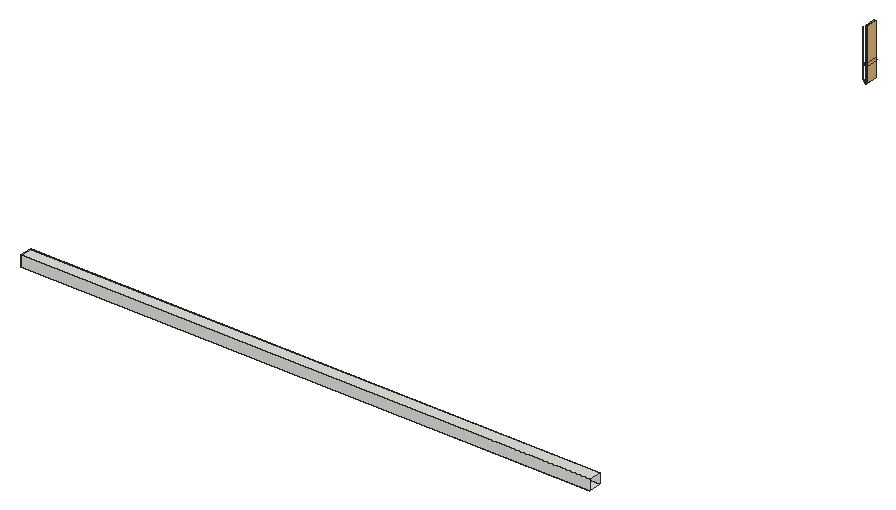
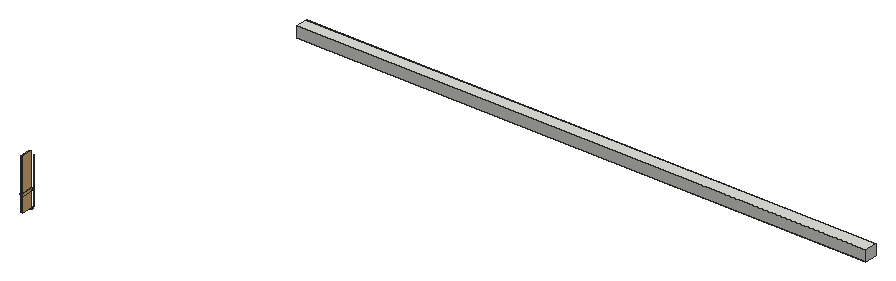
# SketchUp Ruby script. Lengths in inches.
U = 1.inch
M = Sketchup.active_model
def pt(a) = Geom::Point3d.new(a.map { |v| v * U })
def face(e, loops, mat)
  f = e.add_face(loops[0].map { |a| pt(a) })
  loops[1..].each { |l| e.add_face(l.map { |a| pt(a) }).erase! }
  f.material = f.back_material = mat if mat
  f
end
# faces: each face lists its corners as indices into pts; further lists are holes
def faces(e, pts, list, mat = nil) = list.each { |f| face(e, (f[0].is_a?(Array) ? f : [f]).map { |l| l.map { |i| pts[i] } }, mat) }
# xy, xz, yz: faces in a plane at the given z, y or x. An outline is a flat list of corners, or four numbers for a rectangle; further outlines are holes
def ring(l) = l.size == 4 ? [[l[0], l[1]], [l[2], l[1]], [l[2], l[3]], [l[0], l[3]]] : l.each_slice(2).to_a
def flat(e, list, mat, &to3) = list.each { |f| face(e, (f[0].is_a?(Array) ? f : [f]).map { |l| ring(l).map { |u, v| to3.(u, v) } }, mat) }
def xy(e, z, list, mat = nil) = flat(e, list, mat) { |x, y| [x, y, z] }
def xz(e, y, list, mat = nil) = flat(e, list, mat) { |x, z| [x, y, z] }
def yz(e, x, list, mat = nil) = flat(e, list, mat) { |y, z| [x, y, z] }
def lines(e, pts, list) = list.each { |a, b| e.add_line(pt(pts[a]), pt(pts[b])) }
# prism: a flat outline (further loops are holes) pulled along v
def prism(e, loops, v, mat = nil)
  f = face(e, loops, mat); d = Geom::Vector3d.new(v.map { |x| x * U })
  f.pushpull(f.normal.samedirection?(d) ? d.length : -d.length)
end
def box(e, o, s, mat = nil) = prism(e, [[o, [o[0] + s[0], o[1], o[2]], [o[0] + s[0], o[1] + s[1], o[2]], [o[0], o[1] + s[1], o[2]]]], [0, 0, s[2]], mat)
def at(x, y, z, deg = 0) = Geom::Transformation.translation(pt([x, y, z])) * Geom::Transformation.rotation(ORIGIN, Z_AXIS, deg.degrees)
def axes(o, x, y, z) = Geom::Transformation.new([*x, 0, *y, 0, *z, 0, *pt(o).to_a, 1])
def part(name) = M.definitions.add(name)
# library, detail: a bought-in or finely detailed component or shape, given as its bounding box
def library(name, o, s) = part(name).tap { |d| box(d.entities, o, s) }
def detail(e, o, s) = box(e.add_group.entities, o, s)
def put(e, d, t, mat = nil) = e.add_instance(d, t).tap { |i| i.material = mat if mat }
def group(e, t, mat = nil) = e.add_group.tap { |g| g.transformation = t; g.material = mat if mat }.entities
root = M.entities
M.materials.add("Material \#1").color = [140, 140, 140]
c1 = library("3DGeom~4_Defintion",[-18.02,-499.97,-221.16],[36.04,1000,262.12])
c2 = part("3DGeom~5_Defintion")
xy(c2.entities,-225.24,[[-0.79,-499.98,-2.33,-499.64,7.45,-496.14],[-0.79,-499.98,7.45,-496.14,1.58,-499.88],[1.58,-499.88,7.45,-496.14,3.84,-499.16],[-2.33,-499.64,7.4,-485.75,7.45,-496.14],[3.84,-499.16,7.45,-496.14,5.85,-497.89],
  [7.45,-496.14,7.4,-485.75,8.24,-487.08],[7.45,-496.14,8.24,-487.08,8.96,-489.34],[7.45,-496.14,8.96,-489.34,9.0625,-491.71],[7.45,-496.14,9.0625,-491.71,8.55,-494.03],[-7.4,-496.08,-8.24,-494.76,2.32,-482.2],
  [-8.24,-494.76,-8.96,-492.5,2.32,-482.2],[-8.96,-492.5,-9.0625,-490.125,2.32,-482.2],[-9.0625,-490.125,-8.55,-487.81,2.32,-482.2],[-8.55,-487.81,-7.45,-485.7,2.32,-482.2],[-7.45,-485.7,-5.85,-483.95,2.32,-482.2],
  [-5.85,-483.95,-3.84,-482.68,2.32,-482.2],[-3.84,-482.68,-1.58,-481.96,2.32,-482.2],[2.32,-482.2,-1.58,-481.96,0.79,-481.86],[0,481.82,-2.35,482.13,-6.92,496.71],[0,481.82,-6.92,496.71,1.55,482.04],
  [-2.35,482.13,-4.55,483.04,-6.92,496.71],[-4.55,483.04,-6.43,484.49,-6.92,496.71],[-6.43,484.49,-7.88,486.37,-6.92,496.71],[6.92,485.12,-1.55,499.8125,7.88,495.47],[6.92,485.12,7.88,495.47,7.88,486.37],
  [-7.88,486.37,-8.79,488.57,-6.92,496.71],[7.88,486.37,7.88,495.47,8.79,488.57],[-8.79,488.57,-9.1,490.92,-6.92,496.71],[8.79,488.57,7.88,495.47,9.1,490.92],[-9.1,490.92,-8.79,493.28,-6.92,496.71],
  [9.1,490.92,7.88,495.47,8.79,493.28],[-8.79,493.28,-7.88,495.47,-6.92,496.71],[7.88,495.47,-1.55,499.8125,0,500.02],[7.88,495.47,0,500.02,2.35,499.71],[7.88,495.47,2.35,499.71,4.55,498.8],
  [7.88,495.47,4.55,498.8,6.43,497.35]],"Material \#1")
xy(c2.entities,-221.57,[[-2.33,-499.64,-5.22,-498.37,7.4,-485.75],[-5.22,-498.37,-7.4,-496.08,5.22,-483.47],[-5.22,-498.37,5.22,-483.47,7.4,-485.75],[-7.4,-496.08,2.32,-482.2,5.22,-483.47],[1.55,482.04,-6.92,496.71,-4.55,498.8],
  [1.55,482.04,-4.55,498.8,4.55,483.04],[4.55,483.04,-4.55,498.8,-1.55,499.8125],[4.55,483.04,-1.55,499.8125,6.92,485.12]],"Material \#1")
xy(c2.entities,38.05,[[-2.33,-499.64,7.4,-485.75,-5.22,-498.37],[-5.22,-498.37,5.22,-483.47,-7.4,-496.08],[-5.22,-498.37,7.4,-485.75,5.22,-483.47],[-7.4,-496.08,5.22,-483.47,2.32,-482.2],[1.55,482.04,-4.55,498.8,-6.92,496.71],
  [1.55,482.04,4.55,483.04,-4.55,498.8],[4.55,483.04,-1.55,499.8125,-4.55,498.8],[4.55,483.04,6.92,485.12,-1.55,499.8125]],"Material \#1")
xy(c2.entities,41.72,[[-0.79,-499.98,7.45,-496.14,-2.33,-499.64],[-0.79,-499.98,1.58,-499.88,7.45,-496.14],[1.58,-499.88,3.84,-499.16,7.45,-496.14],[-2.33,-499.64,7.45,-496.14,7.4,-485.75],[3.84,-499.16,5.85,-497.89,7.45,-496.14],
  [7.45,-496.14,8.24,-487.08,7.4,-485.75],[7.45,-496.14,8.55,-494.03,9.0625,-491.71],[7.45,-496.14,8.96,-489.34,8.24,-487.08],[7.45,-496.14,9.0625,-491.71,8.96,-489.34],[-7.4,-496.08,2.32,-482.2,-8.24,-494.76],
  [-8.24,-494.76,2.32,-482.2,-8.96,-492.5],[-8.96,-492.5,2.32,-482.2,-9.0625,-490.125],[-9.0625,-490.125,2.32,-482.2,-8.55,-487.81],[-8.55,-487.81,2.32,-482.2,-7.45,-485.7],[-7.45,-485.7,2.32,-482.2,-5.85,-483.95],
  [-5.85,-483.95,2.32,-482.2,-3.84,-482.68],[-3.84,-482.68,2.32,-482.2,-1.58,-481.96],[2.32,-482.2,0.79,-481.86,-1.58,-481.96],[0,481.82,-6.92,496.71,-2.35,482.13],[0,481.82,1.55,482.04,-6.92,496.71],
  [-2.35,482.13,-6.92,496.71,-4.55,483.04],[-4.55,483.04,-6.92,496.71,-6.43,484.49],[-6.43,484.49,-6.92,496.71,-7.88,486.37],[6.92,485.12,7.88,495.47,-1.55,499.8125],[6.92,485.12,7.88,486.37,7.88,495.47],
  [-7.88,486.37,-6.92,496.71,-8.79,488.57],[7.88,486.37,8.79,488.57,7.88,495.47],[-8.79,488.57,-6.92,496.71,-9.1,490.92],[8.79,488.57,9.1,490.92,7.88,495.47],[-9.1,490.92,-6.92,496.71,-8.79,493.28],
  [9.1,490.92,8.79,493.28,7.88,495.47],[-8.79,493.28,-6.92,496.71,-7.88,495.47],[7.88,495.47,0,500.02,-1.55,499.8125],[7.88,495.47,2.35,499.71,0,500.02],[7.88,495.47,4.55,498.8,2.35,499.71],
  [7.88,495.47,6.43,497.35,4.55,498.8]],"Material \#1")
c3 = part("3DGeom~10_Defintion")
yz(c3.entities,-68.96,[[-797.08,-844.83,-797.08,-827.59,-922.41,-827.59],[-922.41,-844.83,-797.08,-844.83,-922.41,-827.59]],"Material \#1")
yz(c3.entities,68.97,[[-922.41,-844.83,-797.08,-827.59,-797.08,-844.83],[-922.41,-844.83,-922.41,-827.59,-797.08,-827.59],[-797.08,137.93,-922.41,155.17,-797.08,155.17],[-922.41,137.93,-922.41,155.17,-797.08,137.93]],"Material \#1")
p = [[-15.8,-989.55,-844.83],[-15.8,-989.55,-827.59],[0,-991.38,-827.59],[0,-991.38,-844.83],[15.8,-989.55,-827.59],[15.8,-989.55,-844.83],
  [-30.32,-984.36,-844.83],[-30.32,-984.36,-827.59],[30.31,-984.36,-827.59],[30.31,-984.36,-844.83],[-43.12,-976.21,-844.83],[-43.12,-976.21,-827.59],
  [43.12,-976.21,-827.59],[43.12,-976.21,-844.83],[-53.81,-965.53,-844.83],[-53.81,-965.53,-827.59],[53.8,-965.53,-827.59],[53.8,-965.53,-844.83],
  [-61.95,-952.73,-844.83],[-61.95,-952.73,-827.59],[53.8,-965.53,-827.59],[61.95,-952.73,-827.59],[61.95,-952.73,-844.83],[-67.15,-938.21,-844.83],
  [-67.15,-938.21,-827.59],[67.14,-938.21,-827.59],[67.14,-938.21,-844.83],[-68.96,-922.41,-844.83],[-68.96,-922.41,-827.59],[67.14,-938.21,-827.59],
  [68.97,-922.41,-827.59],[68.97,-922.41,-844.83],[-69.1,-794.86,-844.83],[-69.1,-794.86,-827.59],[-68.96,-797.08,-827.59],[-68.96,-797.08,-844.83],
  [68.97,-797.08,-844.83],[68.97,-797.08,-827.59],[69.11,-794.71,-827.59],[69.11,-794.71,-844.83],[-69.48,-792.73,-844.83],[-69.48,-792.73,-827.59],
  [69.53,-792.51,-827.59],[69.53,-792.51,-844.83],[-70.14,-790.6875,-844.83],[-70.14,-790.6875,-827.59],[70.24,-790.48,-827.59],[70.24,-790.48,-844.83],
  [-71.08,-788.73,-844.83],[-71.08,-788.73,-827.59],[71.22,-788.57,-827.59],[71.22,-788.57,-844.83],[-72.32,-786.86,-844.83],[-72.32,-786.86,-827.59],
  [72.47,-786.78,-827.59],[72.47,-786.78,-844.83],[-73.8,-785.17,-844.83],[-73.8,-785.17,-827.59],[74,-785.04,-827.59],[74,-785.04,-844.83],
  [-75.96,-783.21,-844.83],[-75.96,-783.21,-827.59],[74,-785.04,-827.59],[75.76,-783.39,-827.59],[75.76,-783.39,-844.83],[86.625,-772.95,-827.59],
  [86.61,-772.96,-844.83],[-86.89,-773.25,-844.83],[-86.89,-773.25,-827.59],[-75.96,-783.21,-844.83],[-96.66,-761.8,-844.83],[-96.66,-761.8,-827.59],
  [86.625,-772.95,-827.59],[86.63,-772.94,-844.83],[86.61,-772.96,-844.83],[86.625,-772.95,-827.59],[86.62,-772.95,-827.59],[86.62,-772.95,-827.59],
  [96.31,-761.375,-827.59],[96.31,-761.375,-844.83],[86.63,-772.94,-844.83],[86.625,-772.95,-827.59],[86.62,-772.95,-827.59],[-104.96,-749.18,-844.83],
  [-104.96,-749.18,-827.59],[-96.66,-761.8,-827.59],[-96.66,-761.8,-844.83],[96.31,-761.375,-827.59],[104.62,-748.77,-827.59],[104.62,-748.77,-844.83],
  [-111.64,-735.52,-844.83],[-111.64,-735.52,-827.59],[111.39,-735.21,-827.59],[111.39,-735.21,-844.83],[-116.49,-721.23,-844.83],[-116.49,-721.23,-827.59],
  [116.4375,-720.78,-827.59],[116.4375,-720.78,-844.83],[-119.64,-705.62,-844.83],[-119.64,-705.62,-827.59],[119.6,-705.57,-827.59],[119.6,-705.57,-844.83],
  [-120.6875,-689.65,-844.83],[-120.6875,-689.65,-827.59],[120.69,-689.65,-827.59],[120.69,-689.65,-844.83],[-117.5,-662,-844.83],[-117.5,-662,-827.59],
  [117.5,-662,-827.59],[117.5,-662,-844.83],[-108.41,-636.61,-844.83],[-108.41,-636.61,-827.59],[117.5,-662,-844.83],[108.41,-636.61,-827.59],
  [108.41,-636.61,-844.83],[-93.91,-613.95,-844.83],[-93.91,-613.95,-827.59],[-108.41,-636.61,-827.59],[108.41,-636.61,-844.83],[94.16,-614.19,-827.59],
  [94.16,-614.19,-844.83],[94.16,-614.19,-827.59],[75.46,-595.5,-827.59],[75.46,-595.5,-844.83],[-75.46,-595.5,-844.83],[-75.46,-595.5,-827.59],
  [-93.91,-613.95,-827.59],[-93.91,-613.95,-827.59],[-93.91,-613.95,-844.83],[-53.05,-581.24,-844.83],[-53.05,-581.24,-827.59],[-75.46,-595.5,-827.59],
  [-75.46,-595.5,-844.83],[53.05,-581.24,-827.59],[53.05,-581.24,-844.83],[-27.65,-572.16,-844.83],[-27.65,-572.16,-827.59],[-53.05,-581.24,-827.59],
  [-53.05,-581.24,-844.83],[27.66,-572.16,-827.59],[27.66,-572.16,-844.83],[0,-568.97,-844.83],[0,-568.97,-827.59],[-27.65,-572.16,-827.59],
  [-27.65,-572.16,-844.83],[0,-568.97,-844.83],[-15.8,-989.55,155.17],[0,-991.38,155.17],[0,-991.38,137.93],[-15.8,-989.55,137.93],
  [15.8,-989.55,155.17],[15.8,-989.55,137.93],[-30.32,-984.36,155.17],[-30.32,-984.36,137.93],[30.31,-984.36,155.17],[30.31,-984.36,137.93],
  [-43.125,-976.22,155.17],[-43.125,-976.22,137.93],[43.12,-976.22,155.17],[43.12,-976.22,137.93],[-53.81,-965.53,155.17],[-53.81,-965.53,137.93],
  [53.8,-965.53,155.17],[53.8,-965.53,137.93],[-61.96,-952.73,155.17],[-61.95,-952.73,137.93],[61.95,-952.73,155.17],[61.95,-952.73,137.93],
  [53.8,-965.53,137.93],[-67.15,-938.21,155.17],[-67.15,-938.21,137.93],[67.14,-938.21,155.17],[67.14,-938.21,137.93],[-68.96,-922.41,155.17],
  [-68.96,-922.41,137.93],[68.97,-922.41,155.17],[68.97,-922.41,137.93],[67.14,-938.21,137.93],[-68.97,-797.08,155.17],[-68.97,-797.08,137.93],
  [-69.1,-794.86,155.17],[-69.1,-794.86,137.93],[68.97,-797.08,155.17],[69.11,-794.71,155.17],[69.11,-794.71,137.93],[68.97,-797.08,137.93],
  [-69.48,-792.73,155.17],[-69.48,-792.73,137.93],[69.53,-792.51,155.17],[69.53,-792.51,137.93],[-70.14,-790.6875,155.17],[-70.14,-790.6875,137.93],
  [70.24,-790.48,155.17],[70.24,-790.48,137.93],[-71.08,-788.73,155.17],[-71.08,-788.73,137.93],[71.22,-788.57,155.17],[71.22,-788.57,137.93],
  [-72.32,-786.86,155.17],[-72.32,-786.86,137.93],[72.47,-786.78,155.17],[72.47,-786.78,137.93],[-73.8,-785.17,155.17],[-73.8,-785.17,137.93],
  [74,-785.04,155.17],[74,-785.04,137.93],[-75.96,-783.21,155.17],[-75.96,-783.21,137.93],[75.76,-783.39,155.17],[75.76,-783.39,137.93],
  [74,-785.04,137.93],[86.61,-772.96,155.17],[86.625,-772.95,137.93],[-86.88,-773.25,155.17],[-75.96,-783.21,155.17],[-86.88,-773.25,137.93],
  [-96.66,-761.8,155.17],[-96.66,-761.8,137.93],[86.63,-772.94,155.17],[86.625,-772.95,137.93],[86.61,-772.96,155.17],[86.62,-772.95,137.93],
  [86.625,-772.95,137.93],[96.31,-761.375,155.17],[96.31,-761.375,137.93],[86.62,-772.95,137.93],[86.63,-772.94,155.17],[86.62,-772.95,137.93],
  [86.625,-772.95,137.93],[-104.96,-749.18,155.17],[-96.66,-761.8,155.17],[-96.66,-761.8,137.93],[-104.96,-749.18,137.93],[104.62,-748.77,155.17],
  [104.62,-748.77,137.93],[96.31,-761.375,137.93],[-111.64,-735.52,155.17],[-111.64,-735.52,137.93],[111.39,-735.21,155.17],[111.39,-735.21,137.93],
  [-116.49,-721.23,155.17],[-116.49,-721.23,137.93],[116.4375,-720.78,155.17],[116.4375,-720.78,137.93],[-119.64,-705.62,155.17],[-119.64,-705.62,137.93],
  [119.6,-705.57,155.17],[119.6,-705.57,137.93],[-120.6875,-689.65,155.17],[-120.6875,-689.65,137.93],[120.69,-689.65,155.17],[120.69,-689.65,137.93],
  [-117.5,-662,155.17],[-117.5,-662,137.93],[117.5,-662,155.17],[117.5,-662,137.93],[-108.41,-636.61,155.17],[-108.41,-636.61,137.93],
  [117.5,-662,155.17],[108.41,-636.61,155.17],[108.41,-636.61,137.93],[-93.91,-613.95,155.17],[-108.41,-636.61,137.93],[-93.91,-613.95,137.93],
  [108.41,-636.61,155.17],[94.16,-614.19,155.17],[94.16,-614.19,137.93],[75.46,-595.5,155.17],[75.46,-595.5,137.93],[94.16,-614.19,137.93],
  [-75.46,-595.5,155.17],[-93.91,-613.95,155.17],[-93.91,-613.95,137.93],[-75.46,-595.5,137.93],[-53.05,-581.24,155.17],[-75.46,-595.5,155.17],
  [-75.46,-595.5,137.93],[-53.05,-581.24,137.93],[53.05,-581.24,155.17],[53.05,-581.24,137.93],[-27.65,-572.16,155.17],[-53.05,-581.24,155.17],
  [-53.05,-581.24,137.93],[-27.65,-572.16,137.93],[27.65,-572.16,155.17],[27.65,-572.16,137.93],[0,-568.97,155.17],[-27.65,-572.16,155.17],
  [-27.65,-572.16,137.93],[0,-568.97,137.93],[0,-568.97,155.17]]
faces(c3.entities,p,[[0,1,2],[2,3,0],[3,2,4],[4,5,3],[6,7,1],[1,0,6],[5,4,8],[8,9,5],
  [10,11,7],[7,6,10],[9,8,12],[12,13,9],[14,15,11],[11,10,14],[13,12,16],[16,17,13],
  [18,19,15],[15,14,18],[17,20,21],[21,22,17],[23,24,19],[19,18,23],[22,21,25],[25,26,22],
  [27,28,24],[24,23,27],[26,29,30],[30,31,26],[32,33,34],[34,35,32],[36,37,38],[38,39,36],
  [40,41,33],[33,32,40],[39,38,42],[42,43,39],[44,45,41],[41,40,44],[43,42,46],[46,47,43],
  [48,49,45],[45,44,48],[47,46,50],[50,51,47],[52,53,49],[49,48,52],[51,50,54],[54,55,51],
  [56,57,53],[53,52,56],[55,54,58],[58,59,55],[60,61,57],[57,56,60],[59,62,63],[63,64,59],
  [64,63,65],[65,66,64],[67,68,61],[61,69,67],[70,71,68],[68,67,70],[72,73,66],[74,75,76],
  [73,77,78],[78,79,73],[80,81,82],[83,84,85],[85,86,83],[79,87,88],[88,89,79],[90,91,84],
  [84,83,90],[89,88,92],[92,93,89],[94,95,91],[91,90,94],[93,92,96],[96,97,93],[98,99,95],
  [95,94,98],[97,96,100],[100,101,97],[102,103,99],[99,98,102],[101,100,104],[104,105,101],[106,107,103],
  [103,102,106],[105,104,108],[108,109,105],[110,111,107],[107,106,110],[112,108,113],[113,114,112],[115,116,117],
  [117,110,115],[118,113,119],[119,120,118],[120,121,122],[122,123,120],[124,125,126],[127,128,124],[129,130,131],
  [131,132,129],[123,122,133],[133,134,123],[135,136,137],[137,138,135],[134,133,139],[139,140,134],[141,142,143],
  [143,144,141],[140,139,142],[142,145,140],[146,147,148],[148,149,146],[147,150,151],[151,148,147],[152,146,149],
  [149,153,152],[150,154,155],[155,151,150],[156,152,153],[153,157,156],[154,158,159],[159,155,154],[160,156,157],
  [157,161,160],[158,162,163],[163,159,158],[164,160,161],[161,165,164],[162,166,167],[167,168,162],[169,164,165],
  [165,170,169],[166,171,172],[172,167,166],[173,169,170],[170,174,173],[171,175,176],[176,177,171],[178,173,174],
  [174,179,178],[180,178,179],[179,181,180],[182,183,184],[184,185,182],[186,180,181],[181,187,186],[183,188,189],
  [189,184,183],[190,186,187],[187,191,190],[188,192,193],[193,189,188],[194,190,191],[191,195,194],[192,196,197],
  [197,193,192],[198,194,195],[195,199,198],[196,200,201],[201,197,196],[202,198,199],[199,203,202],[200,204,205],
  [205,201,200],[206,202,203],[203,207,206],[204,208,209],[209,210,204],[208,211,212],[212,209,208],[213,214,207],
  [207,215,213],[216,213,215],[215,217,216],[211,218,219],[220,221,222],[218,223,224],[224,225,218],[226,227,228],
  [229,230,231],[231,232,229],[223,233,234],[234,235,223],[236,229,232],[232,237,236],[233,238,239],[239,234,233],
  [240,236,237],[237,241,240],[238,242,243],[243,239,238],[244,240,241],[241,245,244],[242,246,247],[247,243,242],
  [248,244,245],[245,249,248],[246,250,251],[251,247,246],[252,248,249],[249,253,252],[250,254,255],[255,251,250],
  [256,252,253],[253,257,256],[258,259,260],[260,255,258],[261,256,262],[262,263,261],[264,265,266],[266,260,264],
  [265,267,268],[268,269,265],[270,271,272],[272,273,270],[274,275,276],[276,277,274],[267,278,279],[279,268,267],
  [280,281,282],[282,283,280],[278,284,285],[285,279,278],[286,287,288],[288,289,286],[284,290,289],[289,285,284]],"Material \#1")
c4 = library("3DGeom~12_Defintion",[-95.68,-755.75,-830.03],[191.36,191.37,1000])
c5 = library("3DGeom~13_Defintion",[-84.91,-744.98,-830.03],[169.82,169.83,1000])
xy(root,173.3125,[[25.395,31.35,122.041,33.481]])
xy(root,175.125,[[25.395,31.35,122.041,33.481]])
xy(root,193.919,[[101.369,115.812,101.417,115.812,101.369,116.097],[101.417,115.812,101.417,116.097,101.369,116.097]],"Material \#1")
xz(root,31.35,[[25.395,173.3125,122.041,175.125]])
xz(root,33.481,[[25.395,173.3125,122.041,175.125]])
xz(root,115.812,[[101.393,193.557,101.347,193.564,101.393,193.565],[101.393,193.557,101.393,193.565,101.436,193.572],[101.393,193.557,101.436,193.572,101.438,193.564],[101.347,193.564,101.305,193.585,101.349,193.572],[101.347,193.564,101.349,193.572,101.393,193.565],
  [101.438,193.564,101.436,193.572,101.477,193.591],[101.438,193.564,101.477,193.591,101.481,193.585],[101.349,193.572,101.305,193.585,101.308,193.591],[101.305,193.585,101.269,193.618,101.308,193.591],[101.481,193.585,101.477,193.591,101.512,193.623],
  [101.481,193.585,101.512,193.623,101.517,193.618],[101.308,193.591,101.269,193.618,101.273,193.623],[101.269,193.618,101.241,193.66,101.273,193.623],[101.517,193.618,101.512,193.623,101.539,193.664],[101.517,193.618,101.539,193.664,101.545,193.66],
  [101.273,193.623,101.241,193.66,101.247,193.664],[101.241,193.66,101.223,193.71,101.247,193.664],[101.545,193.66,101.539,193.664,101.556,193.712],[101.545,193.66,101.556,193.712,101.562,193.71],[101.247,193.664,101.223,193.71,101.23,193.712],
  [101.223,193.71,101.217,193.764,101.23,193.712],[101.562,193.71,101.556,193.712,101.562,193.764],[101.562,193.71,101.562,193.764,101.568,193.764],[101.23,193.712,101.217,193.764,101.224,193.764],[101.217,193.764,101.223,193.818,101.224,193.764],
  [101.224,193.764,101.223,193.818,101.23,193.816],[101.562,193.764,101.556,193.816,101.568,193.764],[101.568,193.764,101.556,193.816,101.562,193.818],[101.23,193.816,101.223,193.818,101.241,193.868],[101.23,193.816,101.241,193.868,101.247,193.864],
  [101.556,193.816,101.539,193.864,101.562,193.818],[101.562,193.818,101.539,193.864,101.545,193.868],[101.247,193.864,101.241,193.868,101.269,193.91],[101.247,193.864,101.269,193.91,101.273,193.905],[101.539,193.864,101.512,193.905,101.545,193.868],
  [101.545,193.868,101.512,193.905,101.517,193.91],[101.273,193.905,101.269,193.91,101.305,193.943],[101.273,193.905,101.305,193.943,101.308,193.937],[101.512,193.905,101.477,193.937,101.517,193.91],[101.517,193.91,101.477,193.937,101.481,193.943],
  [101.308,193.937,101.305,193.943,101.347,193.964],[101.308,193.937,101.347,193.964,101.349,193.956],[101.477,193.937,101.436,193.956,101.481,193.943],[101.481,193.943,101.436,193.956,101.438,193.964],[101.349,193.956,101.347,193.964,101.393,193.971],
  [101.349,193.956,101.393,193.971,101.393,193.963],[101.436,193.956,101.393,193.963,101.438,193.964],[101.393,193.963,101.393,193.971,101.438,193.964]],"Material \#1")
xz(root,115.821,[[101.393,193.094,101.295,193.149,101.49,193.149],[101.393,193.094,101.338,193.109,101.295,193.149],[101.393,193.094,101.364,193.098,101.338,193.109],[101.338,193.109,101.315,193.126,101.295,193.149],[101.49,193.149,101.172,193.729,101.239,193.619],
  [101.49,193.149,101.263,193.545,101.172,193.729],[101.295,193.149,101.268,193.523,101.268,193.529],[101.295,193.149,101.268,193.529,101.49,193.149],[101.295,193.149,101.271,193.207,101.268,193.523],[101.295,193.149,101.281,193.177,101.271,193.207],
  [101.49,193.149,101.306,193.555,101.348,193.538],[101.271,193.207,101.268,193.241,101.268,193.523],[101.263,193.545,101.26,193.55,101.172,193.729],[101.26,193.55,101.257,193.555,101.172,193.729],[101.257,193.555,101.214,193.607,101.172,193.729],
  [101.257,193.555,101.253,193.559,101.214,193.607],[101.253,193.559,101.232,193.582,101.214,193.607],[101.214,193.607,101.186,193.664,101.172,193.729],[101.214,193.607,101.199,193.634,101.186,193.664],[101.239,193.619,101.172,193.729,101.216,193.662],
  [101.216,193.662,101.172,193.729,101.201,193.711],[101.186,193.664,101.177,193.696,101.172,193.729],[101.201,193.711,101.172,193.729,101.196,193.764],[101.172,193.729,101.17,193.764,101.176,193.824],[101.172,193.729,101.176,193.824,101.219,193.929],
  [101.172,193.729,101.201,193.817,101.196,193.764],[101.172,193.729,101.219,193.929,101.201,193.817],[101.201,193.817,101.219,193.929,101.216,193.866],[101.176,193.824,101.192,193.88,101.219,193.929],[101.216,193.866,101.219,193.929,101.239,193.909],
  [101.239,193.909,101.219,193.929,101.27,193.945],[101.219,193.929,101.253,193.969,101.295,194.001],[101.219,193.929,101.295,194.001,101.393,194.027],[101.219,193.929,101.306,193.973,101.27,193.945],[101.219,193.929,101.393,194.027,101.306,193.973],
  [101.306,193.973,101.393,194.027,101.348,193.99],[101.348,193.99,101.393,194.027,101.393,193.996],[101.295,194.001,101.342,194.02,101.393,194.027]],"Material \#1")
xz(root,115.852,[[101.393,190.763,101.29,190.774,101.393,190.775],[101.29,190.774,101.193,190.805,101.291,190.785],[101.29,190.774,101.291,190.785,101.393,190.775],[101.291,190.785,101.193,190.805,101.196,190.816],[101.193,190.805,101.103,190.856,101.196,190.816],
  [101.196,190.816,101.103,190.856,101.108,190.866],[101.103,190.856,101.023,190.922,101.108,190.866],[101.108,190.866,101.023,190.922,101.03,190.931],[101.023,190.922,100.954,191.004,101.03,190.931],[101.03,190.931,100.954,191.004,100.961,191.012],
  [101.393,190.944,101.359,190.948,101.393,190.956],[101.359,190.948,101.326,190.958,101.36,190.959],[101.359,190.948,101.36,190.959,101.393,190.956],[101.326,190.958,101.297,190.975,101.33,190.969],[101.326,190.958,101.33,190.969,101.36,190.959],
  [101.33,190.969,101.297,190.975,101.302,190.985],[101.297,190.975,101.27,190.997,101.302,190.985],[101.302,190.985,101.27,190.997,101.276,191.006],[101.27,190.997,101.247,191.024,101.276,191.006],[100.954,191.004,100.9,191.093,100.961,191.012],
  [101.276,191.006,101.247,191.024,101.255,191.032],[100.961,191.012,100.9,191.093,100.909,191.099],[101.247,191.024,101.228,191.056,101.255,191.032],[101.255,191.032,101.228,191.056,101.237,191.062],[101.228,191.056,101.214,191.091,101.237,191.062],
  [101.237,191.062,101.214,191.091,101.223,191.095],[101.214,191.091,101.205,191.129,101.223,191.095],[100.9,191.093,100.855,191.204,100.909,191.099],[101.223,191.095,101.205,191.129,101.215,191.131],[100.909,191.099,100.855,191.204,100.864,191.208],
  [101.205,191.129,101.202,191.165,101.215,191.131],[101.215,191.131,101.202,191.165,101.212,191.165],[101.202,191.165,101.205,191.21,101.212,191.165],[101.212,191.165,101.205,191.21,101.215,191.207],[100.855,191.204,100.828,191.319,100.864,191.208],
  [101.215,191.207,101.205,191.21,101.214,191.248],[101.215,191.207,101.214,191.248,101.223,191.244],[100.864,191.208,100.828,191.319,100.838,191.321],[101.223,191.244,101.214,191.248,101.228,191.283],[101.223,191.244,101.228,191.283,101.237,191.277],
  [101.237,191.277,101.228,191.283,101.247,191.314],[101.237,191.277,101.247,191.314,101.255,191.307],[101.255,191.307,101.247,191.314,101.27,191.341],[101.255,191.307,101.27,191.341,101.276,191.332],[100.828,191.319,100.819,191.445,100.838,191.321],
  [100.838,191.321,100.819,191.445,100.828,191.445],[101.276,191.332,101.27,191.341,101.297,191.364],[101.276,191.332,101.297,191.364,101.302,191.353],[101.302,191.353,101.297,191.364,101.326,191.38],[101.302,191.353,101.326,191.38,101.33,191.369],
  [101.33,191.369,101.326,191.38,101.359,191.391],[101.33,191.369,101.359,191.391,101.36,191.379],[101.36,191.379,101.359,191.391,101.393,191.394],[101.36,191.379,101.393,191.394,101.393,191.383],[100.819,191.445,100.819,199.181,100.828,191.445],
  [100.828,191.445,100.819,199.181,100.828,199.181]],"Material \#1")
xz(root,115.882,[[101.393,193.532,101.342,193.54,101.393,193.539],[101.393,193.532,101.393,193.539,101.442,193.547],[101.393,193.532,101.442,193.547,101.444,193.54],[101.393,193.539,101.342,193.54,101.344,193.547],[101.342,193.54,101.294,193.563,101.344,193.547],
  [101.444,193.54,101.442,193.547,101.488,193.57],[101.444,193.54,101.488,193.57,101.491,193.563],[101.344,193.547,101.294,193.563,101.298,193.57],[101.294,193.563,101.254,193.6,101.298,193.57],[101.491,193.563,101.488,193.57,101.527,193.605],
  [101.491,193.563,101.527,193.605,101.532,193.6],[101.298,193.57,101.254,193.6,101.258,193.605],[101.254,193.6,101.222,193.648,101.258,193.605],[101.532,193.6,101.527,193.605,101.558,193.652],[101.532,193.6,101.558,193.652,101.563,193.648],
  [101.258,193.605,101.222,193.648,101.228,193.652],[101.222,193.648,101.203,193.704,101.228,193.652],[101.563,193.648,101.558,193.652,101.577,193.706],[101.563,193.648,101.577,193.706,101.583,193.704],[101.228,193.652,101.203,193.704,101.209,193.706],
  [101.203,193.704,101.196,193.764,101.209,193.706],[101.583,193.704,101.577,193.706,101.583,193.764],[101.583,193.704,101.583,193.764,101.59,193.764],[101.209,193.706,101.196,193.764,101.203,193.764],[101.196,193.764,101.203,193.824,101.203,193.764],
  [101.203,193.764,101.203,193.824,101.209,193.822],[101.583,193.764,101.577,193.822,101.59,193.764],[101.59,193.764,101.577,193.822,101.583,193.824],[101.209,193.822,101.203,193.824,101.222,193.88],[101.209,193.822,101.222,193.88,101.228,193.876],
  [101.577,193.822,101.558,193.876,101.583,193.824],[101.583,193.824,101.558,193.876,101.563,193.88],[101.228,193.876,101.222,193.88,101.254,193.928],[101.228,193.876,101.254,193.928,101.258,193.923],[101.558,193.876,101.527,193.923,101.563,193.88],
  [101.563,193.88,101.527,193.923,101.532,193.928],[101.258,193.923,101.254,193.928,101.294,193.965],[101.258,193.923,101.294,193.965,101.298,193.958],[101.527,193.923,101.488,193.958,101.532,193.928],[101.532,193.928,101.488,193.958,101.491,193.965],
  [101.298,193.958,101.294,193.965,101.342,193.988],[101.298,193.958,101.342,193.988,101.344,193.981],[101.488,193.958,101.442,193.981,101.491,193.965],[101.491,193.965,101.442,193.981,101.444,193.988],[101.344,193.981,101.342,193.988,101.393,193.996],
  [101.344,193.981,101.393,193.996,101.393,193.989],[101.442,193.981,101.393,193.989,101.444,193.988],[101.444,193.988,101.393,193.989,101.393,193.996]],"Material \#1")
xz(root,116.097,[[101.384,193.609,101.374,193.632,101.403,193.632],[101.384,193.609,101.403,193.632,101.412,193.609],[101.374,193.632,101.369,193.64,101.408,193.64],[101.374,193.632,101.408,193.64,101.403,193.632],[101.369,193.64,101.369,193.657,101.408,193.657],
  [101.369,193.64,101.408,193.657,101.408,193.64],[101.369,193.657,101.374,193.665,101.403,193.665],[101.369,193.657,101.403,193.665,101.408,193.657],[101.374,193.665,101.374,193.694,101.412,193.694],[101.374,193.665,101.412,193.694,101.403,193.665],
  [101.374,193.694,101.374,193.721,101.412,193.721],[101.374,193.694,101.412,193.721,101.412,193.694],[101.374,193.721,101.367,193.743,101.419,193.743],[101.374,193.721,101.419,193.743,101.412,193.721],[101.367,193.743,101.367,193.765,101.419,193.765],
  [101.367,193.743,101.419,193.765,101.419,193.743],[101.367,193.765,101.374,193.787,101.412,193.787],[101.367,193.765,101.412,193.787,101.419,193.765],[101.374,193.787,101.369,193.803,101.417,193.803],[101.374,193.787,101.417,193.803,101.412,193.787],
  [101.369,193.803,101.369,193.853,101.417,193.853],[101.369,193.803,101.417,193.853,101.417,193.803],[101.369,193.853,101.375,193.857,101.411,193.857],[101.369,193.853,101.411,193.857,101.417,193.853],[101.375,193.857,101.375,193.865,101.411,193.865],
  [101.375,193.857,101.411,193.865,101.411,193.857],[101.375,193.865,101.369,193.869,101.417,193.869],[101.375,193.865,101.417,193.869,101.411,193.865],[101.369,193.869,101.369,193.919,101.417,193.919],[101.369,193.869,101.417,193.919,101.417,193.869]],"Material \#1")
xz(root,116.128,[[101.393,193.094,101.338,193.109,101.364,193.098],[101.393,193.094,101.448,193.109,101.338,193.109],[101.338,193.109,101.268,193.523,101.271,193.207],[101.338,193.109,101.514,193.207,101.268,193.523],[101.338,193.109,101.271,193.207,101.295,193.149],
  [101.338,193.109,101.295,193.149,101.315,193.126],[101.295,193.149,101.271,193.207,101.281,193.177],[101.514,193.207,101.263,193.545,101.265,193.54],[101.514,193.207,101.265,193.54,101.267,193.534],[101.514,193.207,101.267,193.534,101.268,193.529],
  [101.271,193.207,101.268,193.523,101.268,193.241],[101.514,193.207,101.268,193.529,101.268,193.523],[101.517,193.241,101.239,193.619,101.263,193.545],[101.517,193.241,101.27,193.583,101.239,193.619],[101.517,193.241,101.306,193.555,101.27,193.583],
  [101.517,193.241,101.348,193.538,101.306,193.555],[101.263,193.545,101.172,193.729,101.26,193.55],[101.263,193.545,101.216,193.662,101.172,193.729],[101.263,193.545,101.239,193.619,101.216,193.662],[101.26,193.55,101.172,193.729,101.257,193.555],
  [101.257,193.555,101.172,193.729,101.214,193.607],[101.257,193.555,101.214,193.607,101.253,193.559],[101.253,193.559,101.214,193.607,101.232,193.582],[101.214,193.607,101.172,193.729,101.186,193.664],[101.214,193.607,101.186,193.664,101.199,193.634],
  [101.216,193.662,101.201,193.711,101.172,193.729],[101.186,193.664,101.172,193.729,101.177,193.696],[101.201,193.711,101.196,193.764,101.172,193.729],[101.172,193.729,101.176,193.824,101.17,193.764],[101.172,193.729,101.196,193.764,101.201,193.817],
  [101.172,193.729,101.201,193.817,101.216,193.866],[101.172,193.729,101.216,193.866,101.219,193.929],[101.172,193.729,101.219,193.929,101.176,193.824],[101.176,193.824,101.219,193.929,101.192,193.88],[101.216,193.866,101.239,193.909,101.219,193.929],
  [101.239,193.909,101.27,193.945,101.219,193.929],[101.219,193.929,101.27,193.945,101.306,193.973],[101.219,193.929,101.295,194.001,101.253,193.969],[101.219,193.929,101.306,193.973,101.393,194.027],[101.219,193.929,101.393,194.027,101.295,194.001],
  [101.306,193.973,101.348,193.99,101.393,194.027],[101.348,193.99,101.393,193.996,101.393,194.027],[101.295,194.001,101.393,194.027,101.342,194.02]],"Material \#1")
xz(root,117.355,[[101.172,193.729,101.17,193.764,101.176,193.824],[101.172,193.729,101.176,193.824,101.219,193.929],[101.172,193.729,101.216,193.866,101.201,193.817],[101.172,193.729,101.219,193.929,101.216,193.866],[101.176,193.824,101.192,193.88,101.219,193.929],
  [101.216,193.866,101.219,193.929,101.239,193.909],[101.239,193.909,101.219,193.929,101.27,193.945],[101.219,193.929,101.253,193.969,101.295,194.001],[101.219,193.929,101.295,194.001,101.393,194.027],[101.219,193.929,101.393,194.027,101.306,193.973],
  [101.306,193.973,101.393,194.027,101.348,193.99],[101.348,193.99,101.393,194.027,101.393,193.996],[101.295,194.001,101.342,194.02,101.393,194.027]],"Material \#1")
yz(root,25.395,[[31.35,173.3125,33.481,175.125]])
yz(root,101.369,[[116.097,193.869,115.812,193.919,116.097,193.919]],"Material \#1")
yz(root,101.374,[[116.097,193.665,115.812,193.694,116.097,193.694]],"Material \#1")
p = [[101.329,115.858,191.062],[101.329,115.882,191.062],[101.349,115.882,191.05],[101.349,115.858,191.05],[101.363,115.876,191.074],[101.363,115.851,191.074],
  [101.409,115.849,191.243],[101.409,115.873,191.243],[101.34,115.873,191.126],[101.34,115.849,191.126],[101.327,115.876,191.104],[101.327,115.851,191.104],
  [101.376,115.873,191.096],[101.376,115.849,191.096],[101.446,115.873,191.213],[101.446,115.849,191.213],[101.3125,115.882,191.08],[101.3125,115.858,191.08],
  [101.459,115.876,191.235],[101.459,115.851,191.235],[101.422,115.851,191.265],[101.422,115.876,191.265],[101.473,115.882,191.259],[101.473,115.858,191.259],
  [101.456,115.858,191.277],[101.456,115.882,191.277],[101.437,115.882,191.289],[101.437,115.858,191.289],[101.372,115.812,193.661],[101.369,116.097,193.657],
  [101.369,116.097,193.64],[101.372,115.812,193.636],[101.372,115.812,193.636],[101.369,116.097,193.64],[101.374,116.097,193.632],[101.372,115.812,193.636],
  [101.374,116.097,193.632],[101.384,116.097,193.609],[101.384,115.812,193.609],[101.372,115.812,193.636],[101.374,116.097,193.665],[101.372,115.812,193.661],
  [101.374,115.812,193.694],[101.374,116.097,193.721],[101.37,115.812,193.732],[101.367,115.812,193.754],[101.374,116.097,193.694],[101.374,115.812,193.694],
  [101.37,115.812,193.732],[101.367,116.097,193.743],[101.367,115.812,193.754],[101.37,115.812,193.776],[101.372,115.812,193.661],[101.374,116.097,193.665],
  [101.369,116.097,193.657],[101.367,115.812,193.754],[101.367,116.097,193.743],[101.374,116.097,193.721],[101.37,115.812,193.732],[101.374,116.097,193.721],
  [101.374,116.097,193.694],[101.37,115.812,193.776],[101.367,116.097,193.765],[101.367,116.097,193.743],[101.369,116.097,193.803],[101.369,115.812,193.806],
  [101.371,115.812,193.857],[101.374,116.097,193.787],[101.372,115.812,193.795],[101.369,115.812,193.806],[101.367,116.097,193.765],[101.37,115.812,193.776],
  [101.372,115.812,193.795],[101.371,115.812,193.857],[101.369,116.097,193.853],[101.369,116.097,193.803],[101.369,115.812,193.806],[101.369,116.097,193.803],
  [101.374,116.097,193.787],[101.372,115.812,193.795],[101.374,116.097,193.787],[101.367,116.097,193.765],[101.369,116.097,193.869],[101.371,115.812,193.857],
  [101.369,115.812,193.919],[101.414,115.812,193.862],[101.417,116.097,193.853],[101.411,116.097,193.857],[101.371,115.812,193.857],[101.375,116.097,193.865],
  [101.375,116.097,193.857],[101.371,115.812,193.857],[101.369,116.097,193.869],[101.371,115.812,193.857],[101.369,116.097,193.853],[101.414,115.812,193.862],
  [101.411,116.097,193.865],[101.417,116.097,193.869],[101.414,115.812,193.862]]
faces(root,p,[[0,1,2],[2,3,0],[3,2,4],[4,5,3],[6,7,8],[8,9,6],[9,8,10],[10,11,9],
  [12,13,5],[13,12,14],[14,15,13],[11,10,16],[16,17,11],[17,16,1],[1,0,17],[5,4,12],
  [15,14,18],[18,19,15],[7,6,20],[20,21,7],[19,18,22],[22,23,19],[24,25,26],[26,27,24],
  [27,26,21],[21,20,27],[23,22,25],[25,24,23],[28,29,30],[30,31,28],[32,33,34],[35,36,37],
  [37,38,39],[40,41,42],[43,44,45],[46,47,48],[49,50,51],[52,53,54],[55,56,57],[58,59,60],
  [61,62,63],[64,65,66],[67,68,69],[70,71,72],[73,74,75],[76,77,78],[79,80,81],[82,83,84],
  [85,86,87],[88,89,90],[91,92,89],[93,90,94],[95,96,97],[98,87,96]],"Material \#1")
put(root,c1,axes([101.39,117.36,195.3125],[0.00728,0,0],[0,0,0.0086],[0,0.00681,0]),"Material \#1")
put(root,c2,axes([101.39,117.36,195.3125],[0.00715,0,0],[0,0,0.00844],[0,0.00669,0]),"Material \#1")
put(root,c3,axes([101.39,117.36,195.3125],[0.0019,0,0],[0,0,0.00225],[0,0.00178,0]),"Material \#1")
put(root,c4,axes([101.39,117.36,195.3125],[0.00199,0,0],[0,0,0.00235],[0,0.00186,0]),"Material \#1")
put(root,c5,axes([101.39,117.36,195.3125],[0.00199,0,0],[0,0,0.00235],[0,0.00186,0]),"Material \#1")
